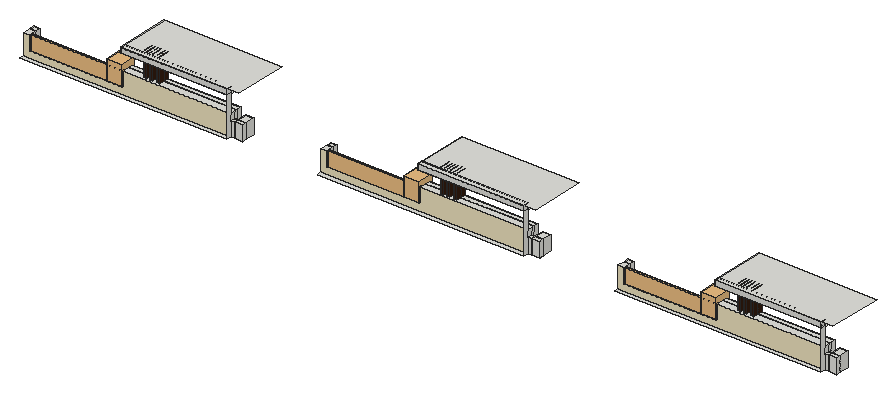
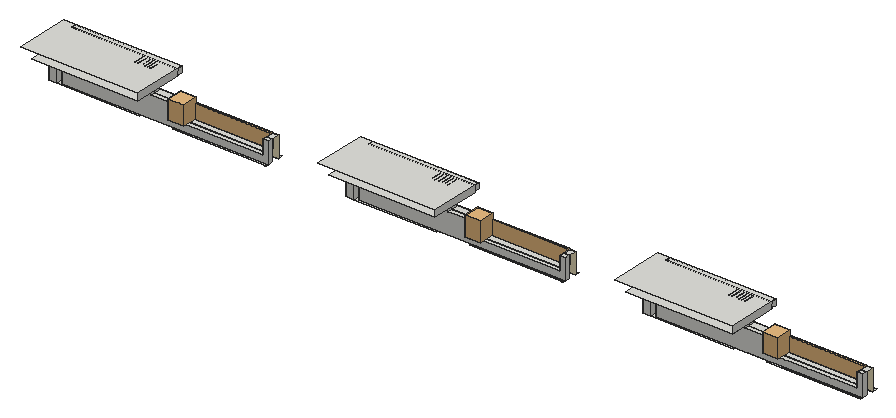
# SketchUp Ruby script. Lengths in inches.
U = 1.inch
M = Sketchup.active_model
def pt(a) = Geom::Point3d.new(a.map { |v| v * U })
def face(e, loops, mat)
  f = e.add_face(loops[0].map { |a| pt(a) })
  loops[1..].each { |l| e.add_face(l.map { |a| pt(a) }).erase! }
  f.material = f.back_material = mat if mat
  f
end
# faces: each face lists its corners as indices into pts; further lists are holes
def faces(e, pts, list, mat = nil) = list.each { |f| face(e, (f[0].is_a?(Array) ? f : [f]).map { |l| l.map { |i| pts[i] } }, mat) }
# xy, xz, yz: faces in a plane at the given z, y or x. An outline is a flat list of corners, or four numbers for a rectangle; further outlines are holes
def ring(l) = l.size == 4 ? [[l[0], l[1]], [l[2], l[1]], [l[2], l[3]], [l[0], l[3]]] : l.each_slice(2).to_a
def flat(e, list, mat, &to3) = list.each { |f| face(e, (f[0].is_a?(Array) ? f : [f]).map { |l| ring(l).map { |u, v| to3.(u, v) } }, mat) }
def xy(e, z, list, mat = nil) = flat(e, list, mat) { |x, y| [x, y, z] }
def xz(e, y, list, mat = nil) = flat(e, list, mat) { |x, z| [x, y, z] }
def yz(e, x, list, mat = nil) = flat(e, list, mat) { |y, z| [x, y, z] }
def lines(e, pts, list) = list.each { |a, b| e.add_line(pt(pts[a]), pt(pts[b])) }
# prism: a flat outline (further loops are holes) pulled along v
def prism(e, loops, v, mat = nil)
  f = face(e, loops, mat); d = Geom::Vector3d.new(v.map { |x| x * U })
  f.pushpull(f.normal.samedirection?(d) ? d.length : -d.length)
end
def box(e, o, s, mat = nil) = prism(e, [[o, [o[0] + s[0], o[1], o[2]], [o[0] + s[0], o[1] + s[1], o[2]], [o[0], o[1] + s[1], o[2]]]], [0, 0, s[2]], mat)
def at(x, y, z, deg = 0) = Geom::Transformation.translation(pt([x, y, z])) * Geom::Transformation.rotation(ORIGIN, Z_AXIS, deg.degrees)
def axes(o, x, y, z) = Geom::Transformation.new([*x, 0, *y, 0, *z, 0, *pt(o).to_a, 1])
def part(name) = M.definitions.add(name)
# library, detail: a bought-in or finely detailed component or shape, given as its bounding box
def library(name, o, s) = part(name).tap { |d| box(d.entities, o, s) }
def detail(e, o, s) = box(e.add_group.entities, o, s)
def put(e, d, t, mat = nil) = e.add_instance(d, t).tap { |i| i.material = mat if mat }
def group(e, t, mat = nil) = e.add_group.tap { |g| g.transformation = t; g.material = mat if mat }.entities
root = M.entities
M.materials.add("[Color D01]").color = [237, 225, 189]
M.materials.add("[Wood Veneer 01]").color = [51, 28, 15]
c1 = library("plant (1)",[-35.72,-28.42,0],[66.31,67.39,84.38])
c2 = library("Glass Railing",[0,0,0],[139.5,4.76,42])
xy(root,524.9375,[[83.125,246.64,593.4375,258.35],[816.6875,246.64,1327,258.35],[1550.25,246.64,2060.5625,258.35],[602.25,258.35,622,270.05],[622,258.35,622.125,270.05],
  [1335.8125,258.35,1355.5625,270.05],[1355.5625,258.35,1355.6875,270.05],[2069.375,258.35,2089.125,270.05],[2089.125,258.35,2089.25,270.05],[593.5,270.05,602.25,270.05,602.25,293.45,396.57,293.45,396.57,289.27,593.5,289.27],
  [602.25,270.05,622,293.45],[622,270.05,622.125,293.45],[1327.0625,270.05,1335.8125,270.05,1335.8125,293.45,1130.14,293.45,1130.14,289.27,1327.0625,289.27],[1335.8125,270.05,1355.5625,293.45],[1355.5625,270.05,1355.6875,293.45],
  [2060.625,270.05,2069.375,270.05,2069.375,293.45,1863.7,293.45,1863.7,289.27,2060.625,289.27],[2069.375,270.05,2089.125,293.45],[2089.125,270.05,2089.25,293.45],[318.81,271.96,322.23,277.39],[1052.37,271.96,1055.8,277.39],
  [1785.93,271.96,1789.36,277.39],[390.12,272.89,393.55,277.39],[1123.68,272.89,1127.11,277.39],[1857.25,272.89,1860.67,277.39],[83.125,277.39,318.81,277.39,318.81,286.21,315.43,286.21,315.43,289.27,83.125,289.27],
  [318.81,277.39,322.23,289.27],[322.23,277.39,322.23,286.21,324.81,286.21,324.81,282.52,328.23,282.52,328.23,286.21,330.81,286.21,330.81,282.52,334.23,282.52,334.23,286.21,336.81,286.21,336.81,282.52,340.23,282.52,340.23,286.21,342.81,286.21,342.81,282.52,346.23,282.52,346.23,286.21,348.81,286.21,348.81,283.46,352.23,283.46,352.23,286.21,354.81,286.21,354.81,283.46,358.23,283.46,358.23,286.21,360.81,286.21,360.81,283.46,364.23,283.46,364.23,286.21,366.81,286.21,366.81,283.46,370.23,283.46,370.23,286.21,372.81,286.21,372.81,283.46,376.23,283.46,376.23,286.21,378.81,286.21,378.81,283.46,382.23,283.46,382.23,286.21,384.81,286.21,384.81,283.46,388.23,283.46,388.23,286.21,390.12,286.21,390.12,277.39],[390.12,277.39,393.55,289.27],[393.55,277.39,593.5,277.39,593.5,289.27,396.57,289.27,396.57,286.21,393.55,286.21],[816.6875,277.39,1052.37,277.39,1052.37,286.21,1049,286.21,1049,289.27,816.6875,289.27],
  [1052.37,277.39,1055.8,289.27],[1055.8,277.39,1055.8,286.21,1058.37,286.21,1058.37,282.52,1061.8,282.52,1061.8,286.21,1064.37,286.21,1064.37,282.52,1067.8,282.52,1067.8,286.21,1070.37,286.21,1070.37,282.52,1073.8,282.52,1073.8,286.21,1076.37,286.21,1076.37,282.52,1079.8,282.52,1079.8,286.21,1082.37,286.21,1082.37,283.46,1085.8,283.46,1085.8,286.21,1088.37,286.21,1088.37,283.46,1091.8,283.46,1091.8,286.21,1094.37,286.21,1094.37,283.46,1097.8,283.46,1097.8,286.21,1100.37,286.21,1100.37,283.46,1103.8,283.46,1103.8,286.21,1106.37,286.21,1106.37,283.46,1109.8,283.46,1109.8,286.21,1112.37,286.21,1112.37,283.46,1115.8,283.46,1115.8,286.21,1118.37,286.21,1118.37,283.46,1121.8,283.46,1121.8,286.21,1123.68,286.21,1123.68,277.39],[1123.68,277.39,1127.11,289.27],[1127.11,277.39,1327.0625,277.39,1327.0625,289.27,1130.14,289.27,1130.14,286.21,1127.11,286.21],[1550.25,277.39,1785.93,277.39,1785.93,286.21,1782.56,286.21,1782.56,289.27,1550.25,289.27],
  [1785.93,277.39,1789.36,289.27],[1789.36,277.39,1789.36,286.21,1791.93,286.21,1791.93,282.52,1795.36,282.52,1795.36,286.21,1797.93,286.21,1797.93,282.52,1801.36,282.52,1801.36,286.21,1803.93,286.21,1803.93,282.52,1807.36,282.52,1807.36,286.21,1809.93,286.21,1809.93,282.52,1813.36,282.52,1813.36,286.21,1815.93,286.21,1815.93,283.46,1819.36,283.46,1819.36,286.21,1821.93,286.21,1821.93,283.46,1825.36,283.46,1825.36,286.21,1827.93,286.21,1827.93,283.46,1831.36,283.46,1831.36,286.21,1833.93,286.21,1833.93,283.46,1837.36,283.46,1837.36,286.21,1839.93,286.21,1839.93,283.46,1843.36,283.46,1843.36,286.21,1845.93,286.21,1845.93,283.46,1849.36,283.46,1849.36,286.21,1851.93,286.21,1851.93,283.46,1855.36,283.46,1855.36,286.21,1857.25,286.21,1857.25,277.39],[1857.25,277.39,1860.67,289.27],[1860.67,277.39,2060.625,277.39,2060.625,289.27,1863.7,289.27,1863.7,286.21,1860.67,286.21],[324.81,282.52,324.81,286.21,322.23,286.21,322.23,289.27,390.12,289.27,390.12,286.21,388.23,286.21,388.23,283.46,384.81,283.46,384.81,286.21,382.23,286.21,382.23,283.46,378.81,283.46,378.81,286.21,376.23,286.21,376.23,283.46,372.81,283.46,372.81,286.21,370.23,286.21,370.23,283.46,366.81,283.46,366.81,286.21,364.23,286.21,364.23,283.46,360.81,283.46,360.81,286.21,358.23,286.21,358.23,283.46,354.81,283.46,354.81,286.21,352.23,286.21,352.23,283.46,348.81,283.46,348.81,286.21,346.23,286.21,346.23,282.52,342.81,282.52,342.81,286.21,340.23,286.21,340.23,282.52,336.81,282.52,336.81,286.21,334.23,286.21,334.23,282.52,330.81,282.52,330.81,286.21,328.23,286.21,328.23,282.52],
  [1058.37,282.52,1058.37,286.21,1055.8,286.21,1055.8,289.27,1123.68,289.27,1123.68,286.21,1121.8,286.21,1121.8,283.46,1118.37,283.46,1118.37,286.21,1115.8,286.21,1115.8,283.46,1112.37,283.46,1112.37,286.21,1109.8,286.21,1109.8,283.46,1106.37,283.46,1106.37,286.21,1103.8,286.21,1103.8,283.46,1100.37,283.46,1100.37,286.21,1097.8,286.21,1097.8,283.46,1094.37,283.46,1094.37,286.21,1091.8,286.21,1091.8,283.46,1088.37,283.46,1088.37,286.21,1085.8,286.21,1085.8,283.46,1082.37,283.46,1082.37,286.21,1079.8,286.21,1079.8,282.52,1076.37,282.52,1076.37,286.21,1073.8,286.21,1073.8,282.52,1070.37,282.52,1070.37,286.21,1067.8,286.21,1067.8,282.52,1064.37,282.52,1064.37,286.21,1061.8,286.21,1061.8,282.52],[1791.93,282.52,1791.93,286.21,1789.36,286.21,1789.36,289.27,1857.25,289.27,1857.25,286.21,1855.36,286.21,1855.36,283.46,1851.93,283.46,1851.93,286.21,1849.36,286.21,1849.36,283.46,1845.93,283.46,1845.93,286.21,1843.36,286.21,1843.36,283.46,1839.93,283.46,1839.93,286.21,1837.36,286.21,1837.36,283.46,1833.93,283.46,1833.93,286.21,1831.36,286.21,1831.36,283.46,1827.93,283.46,1827.93,286.21,1825.36,286.21,1825.36,283.46,1821.93,283.46,1821.93,286.21,1819.36,286.21,1819.36,283.46,1815.93,283.46,1815.93,286.21,1813.36,286.21,1813.36,282.52,1809.93,282.52,1809.93,286.21,1807.36,286.21,1807.36,282.52,1803.93,282.52,1803.93,286.21,1801.36,286.21,1801.36,282.52,1797.93,282.52,1797.93,286.21,1795.36,286.21,1795.36,282.52],[315.43,286.21,318.81,289.27],[393.55,286.21,396.57,289.27],[1049,286.21,1052.37,289.27],
  [1127.11,286.21,1130.14,289.27],[1782.56,286.21,1785.93,289.27],[1860.67,286.21,1863.7,289.27],[83.125,289.27,315.43,293.46],[816.6875,289.27,1049,293.46],
  [1550.25,289.27,1782.56,293.46],[83.125,293.46,315.43,294.83],[816.6875,293.46,1049,294.83],[1550.25,293.46,1782.56,294.83]])
xy(root,541.61,[[97.01,258.35,324.51,277.39],[830.57,258.35,1058.07,277.39],[1564.13,258.35,1791.63,277.39],[97.01,277.39,324.51,289.27],[830.57,277.39,1058.07,289.27],
  [1564.13,277.39,1791.63,289.27]])
xy(root,560.9375,[[593.5,258.35,602.25,270.05],[602.25,258.35,622,270.05],[622,258.35,622.125,270.05],[1327.0625,258.35,1335.8125,270.05],[1335.8125,258.35,1355.5625,270.05],
  [1355.5625,258.35,1355.6875,270.05],[2060.625,258.35,2069.375,270.05],[2069.375,258.35,2089.125,270.05],[2089.125,258.35,2089.25,270.05],[602.25,270.05,622,293.45],
  [622,270.05,622.125,293.45],[1335.8125,270.05,1355.5625,293.45],[1355.5625,270.05,1355.6875,293.45],[2069.375,270.05,2089.125,293.45],[2089.125,270.05,2089.25,293.45]])
xy(root,576.8125,[[83.125,258.35,97.01,277.39],[324.51,258.35,593.5,258.35,593.5,277.39,413.09,277.39,413.09,264.45,405.09,264.45,405.09,277.39,396.02,277.39,396.02,264.45,388.02,264.45,388.02,277.39,381.65,277.39,381.65,264.45,373.65,264.45,373.65,277.39,324.51,277.39],[816.6875,258.35,830.57,277.39],[1058.07,258.35,1327.0625,258.35,1327.0625,277.39,1146.65,277.39,1146.65,264.45,1138.65,264.45,1138.65,277.39,1129.59,277.39,1129.59,264.45,1121.59,264.45,1121.59,277.39,1115.21,277.39,1115.21,264.45,1107.21,264.45,1107.21,277.39,1058.07,277.39],[1550.25,258.35,1564.13,277.39],
  [1791.63,258.35,2060.625,258.35,2060.625,277.39,1880.21,277.39,1880.21,264.45,1872.21,264.45,1872.21,277.39,1863.15,277.39,1863.15,264.45,1855.15,264.45,1855.15,277.39,1848.77,277.39,1848.77,264.45,1840.77,264.45,1840.77,277.39,1791.63,277.39],[83.125,277.39,97.01,289.27],[324.51,277.39,373.65,289.27],[381.65,277.39,388.02,289.27],[396.02,277.39,405.09,289.27],
  [413.09,277.39,593.5,289.27],[816.6875,277.39,830.57,289.27],[1058.07,277.39,1107.21,289.27],[1115.21,277.39,1121.59,289.27],[1129.59,277.39,1138.65,289.27],
  [1146.65,277.39,1327.0625,289.27],[1550.25,277.39,1564.13,289.27],[1791.63,277.39,1840.77,289.27],[1848.77,277.39,1855.15,289.27],[1863.15,277.39,1872.21,289.27],
  [1880.21,277.39,2060.625,289.27]])
xy(root,620.22,[[330.81,258.35,593.5,381.35],[1064.37,258.35,1327.0625,381.35],[1797.93,258.35,2060.625,381.35]])
xy(root,635.84,[[373.65,264.45,381.65,277.39],[388.02,264.45,396.02,277.39],[405.09,264.45,413.09,277.39],[1107.21,264.45,1115.21,277.39],[1121.59,264.45,1129.59,277.39],
  [1138.65,264.45,1146.65,277.39],[1840.77,264.45,1848.77,277.39],[1855.15,264.45,1863.15,277.39],[1872.21,264.45,1880.21,277.39],[373.65,277.39,381.65,289.27],
  [388.02,277.39,396.02,289.27],[405.09,277.39,413.09,289.27],[1107.21,277.39,1115.21,289.27],[1121.59,277.39,1129.59,289.27],[1138.65,277.39,1146.65,289.27],
  [1840.77,277.39,1848.77,289.27],[1855.15,277.39,1863.15,289.27],[1872.21,277.39,1880.21,289.27]])
xy(root,636.53,[[330.81,246.64,622,381.35],[1064.37,246.64,1355.5625,381.35],[1797.93,246.64,2089.125,381.35]])
xz(root,258.35,[[593.4375,524.9375,602.25,524.9375,602.25,560.9375,593.5,560.9375,593.5,576.8125,593.4375,576.8125],[602.25,524.9375,622,560.9375],[622,524.9375,622.125,560.9375],[1327,524.9375,1335.8125,524.9375,1335.8125,560.9375,1327.0625,560.9375,1327.0625,576.8125,1327,576.8125],[1335.8125,524.9375,1355.5625,560.9375],
  [1355.5625,524.9375,1355.6875,560.9375],[2060.5625,524.9375,2069.375,524.9375,2069.375,560.9375,2060.625,560.9375,2060.625,576.8125,2060.5625,576.8125],[2069.375,524.9375,2089.125,560.9375],[2089.125,524.9375,2089.25,560.9375],[593.4375,576.8125,593.5,620.22],
  [1327,576.8125,1327.0625,620.22],[2060.5625,576.8125,2060.625,620.22],[330.81,620.22,593.4375,620.22,593.4375,623.82,593.5,623.82,593.5,636.53,330.81,636.53],[1064.37,620.22,1327,620.22,1327,623.82,1327.0625,623.82,1327.0625,636.53,1064.37,636.53],[1797.93,620.22,2060.5625,620.22,2060.5625,623.82,2060.625,623.82,2060.625,636.53,1797.93,636.53]])
xz(root,258.35,[[83.125,524.9375,593.4375,524.9375,593.4375,576.8125,324.51,576.8125,324.51,541.61,97.01,541.61,97.01,576.8125,83.125,576.8125],[816.6875,524.9375,1327,524.9375,1327,576.8125,1058.07,576.8125,1058.07,541.61,830.57,541.61,830.57,576.8125,816.6875,576.8125],[1550.25,524.9375,2060.5625,524.9375,2060.5625,576.8125,1791.63,576.8125,1791.63,541.61,1564.13,541.61,1564.13,576.8125,1550.25,576.8125]],"[Color D01]")
xz(root,264.45,[[373.65,576.8125,381.65,635.84],[388.02,576.8125,396.02,635.84],[405.09,576.8125,413.09,635.84],[1107.21,576.8125,1115.21,635.84],[1121.59,576.8125,1129.59,635.84],
  [1138.65,576.8125,1146.65,635.84],[1840.77,576.8125,1848.77,635.84],[1855.15,576.8125,1863.15,635.84],[1872.21,576.8125,1880.21,635.84]],"[Wood Veneer 01]")
xz(root,270.05,[[593.5,524.9375,602.25,560.9375],[602.25,524.9375,622.125,560.9375],[1327.0625,524.9375,1335.8125,560.9375],[1335.8125,524.9375,1355.6875,560.9375],[2060.625,524.9375,2069.375,560.9375],
  [2069.375,524.9375,2089.25,560.9375]])
xz(root,277.39,[[83.125,524.9375,593.5,524.9375,593.5,576.8125,413.09,576.8125,413.09,635.84,405.09,635.84,405.09,576.8125,396.02,576.8125,396.02,635.84,388.02,635.84,388.02,576.8125,381.65,576.8125,381.65,635.84,373.65,635.84,373.65,576.8125,324.51,576.8125,324.51,541.61,97.01,541.61,97.01,576.8125,83.125,576.8125],[816.6875,524.9375,1327.0625,524.9375,1327.0625,576.8125,1146.65,576.8125,1146.65,635.84,1138.65,635.84,1138.65,576.8125,1129.59,576.8125,1129.59,635.84,1121.59,635.84,1121.59,576.8125,1115.21,576.8125,1115.21,635.84,1107.21,635.84,1107.21,576.8125,1058.07,576.8125,1058.07,541.61,830.57,541.61,830.57,576.8125,816.6875,576.8125],[1550.25,524.9375,2060.625,524.9375,2060.625,576.8125,1880.21,576.8125,1880.21,635.84,1872.21,635.84,1872.21,576.8125,1863.15,576.8125,1863.15,635.84,1855.15,635.84,1855.15,576.8125,1848.77,576.8125,1848.77,635.84,1840.77,635.84,1840.77,576.8125,1791.63,576.8125,1791.63,541.61,1564.13,541.61,1564.13,576.8125,1550.25,576.8125]])
xz(root,289.27,[[83.125,524.9375,83.125,576.8125,97.01,576.8125,97.01,541.61,324.51,541.61,324.51,576.8125,373.65,576.8125,373.65,635.84,381.65,635.84,381.65,576.8125,388.02,576.8125,388.02,635.84,396.02,635.84,396.02,576.8125,405.09,576.8125,405.09,635.84,413.09,635.84,413.09,576.8125,593.5,576.8125,593.5,524.9375],[816.6875,524.9375,816.6875,576.8125,830.57,576.8125,830.57,541.61,1058.07,541.61,1058.07,576.8125,1107.21,576.8125,1107.21,635.84,1115.21,635.84,1115.21,576.8125,1121.59,576.8125,1121.59,635.84,1129.59,635.84,1129.59,576.8125,1138.65,576.8125,1138.65,635.84,1146.65,635.84,1146.65,576.8125,1327.0625,576.8125,1327.0625,524.9375],[1550.25,524.9375,1550.25,576.8125,1564.13,576.8125,1564.13,541.61,1791.63,541.61,1791.63,576.8125,1840.77,576.8125,1840.77,635.84,1848.77,635.84,1848.77,576.8125,1855.15,576.8125,1855.15,635.84,1863.15,635.84,1863.15,576.8125,1872.21,576.8125,1872.21,635.84,1880.21,635.84,1880.21,576.8125,2060.625,576.8125,2060.625,524.9375]])
xz(root,293.45,[[602.25,524.9375,622,560.9375],[622,524.9375,622.125,560.9375],[1335.8125,524.9375,1355.5625,560.9375],[1355.5625,524.9375,1355.6875,560.9375],[2069.375,524.9375,2089.125,560.9375],
  [2089.125,524.9375,2089.25,560.9375]])
yz(root,83.125,[[277.39,524.9375,289.27,576.8125]])
yz(root,97.01,[[258.35,541.61,277.39,576.8125],[277.39,541.61,289.27,576.8125]])
yz(root,324.51,[[258.35,541.61,277.39,576.8125],[277.39,541.61,289.27,576.8125]])
yz(root,330.81,[[258.35,620.22,258.35,623.82,259.1,623.87,258.35,636.53,246.64,635.84,246.64,636.53,381.35,636.53,381.35,620.22],[247.39,623.17,246.64,635.84,258.35,636.53,258.35,623.82],[258.35,623.82,258.35,636.53,259.1,623.87]])
yz(root,373.65,[[264.45,576.8125,277.39,635.84],[277.39,576.8125,289.27,635.84]])
yz(root,381.65,[[277.39,576.8125,289.27,635.84]])
yz(root,381.65,[[264.45,576.8125,277.39,635.84]],"[Wood Veneer 01]")
yz(root,388.02,[[264.45,576.8125,277.39,635.84],[277.39,576.8125,289.27,635.84]])
yz(root,396.02,[[264.45,576.8125,277.39,635.84],[277.39,576.8125,289.27,635.84]],"[Wood Veneer 01]")
yz(root,405.09,[[264.45,576.8125,277.39,635.84],[277.39,576.8125,289.27,635.84]])
yz(root,413.09,[[264.45,576.8125,277.39,635.84],[277.39,576.8125,289.27,635.84]],"[Wood Veneer 01]")
yz(root,593.4375,[[246.64,524.9375,246.64,635.84,247.39,623.17,258.35,623.82,258.35,524.9375]])
yz(root,593.5,[[270.05,524.9375,277.39,576.8125],[277.39,524.9375,289.27,576.8125],[258.35,560.9375,270.05,576.8125],[247.39,623.17,246.64,635.84,258.35,636.53,258.35,623.82],[258.35,623.82,259.1,623.87,258.35,636.53]])
yz(root,602.25,[[258.35,524.9375,270.05,560.9375],[270.05,524.9375,293.45,560.9375]])
yz(root,622.125,[[258.35,524.9375,270.05,560.9375],[270.05,524.9375,293.45,560.9375]])
yz(root,816.6875,[[277.39,524.9375,289.27,576.8125]])
yz(root,830.57,[[258.35,541.61,277.39,576.8125],[277.39,541.61,289.27,576.8125]])
yz(root,1058.07,[[258.35,541.61,277.39,576.8125],[277.39,541.61,289.27,576.8125]])
yz(root,1064.37,[[258.35,620.22,258.35,623.82,259.1,623.87,258.35,636.53,246.64,635.84,246.64,636.53,381.35,636.53,381.35,620.22],[247.39,623.17,246.64,635.84,258.35,636.53,258.35,623.82],[258.35,623.82,258.35,636.53,259.1,623.87]])
yz(root,1107.21,[[264.45,576.8125,277.39,635.84],[277.39,576.8125,289.27,635.84]])
yz(root,1115.21,[[277.39,576.8125,289.27,635.84]])
yz(root,1115.21,[[264.45,576.8125,277.39,635.84]],"[Wood Veneer 01]")
yz(root,1121.59,[[264.45,576.8125,277.39,635.84],[277.39,576.8125,289.27,635.84]])
yz(root,1129.59,[[264.45,576.8125,277.39,635.84],[277.39,576.8125,289.27,635.84]],"[Wood Veneer 01]")
yz(root,1138.65,[[264.45,576.8125,277.39,635.84],[277.39,576.8125,289.27,635.84]])
yz(root,1146.65,[[264.45,576.8125,277.39,635.84],[277.39,576.8125,289.27,635.84]],"[Wood Veneer 01]")
yz(root,1327,[[246.64,524.9375,246.64,635.84,247.39,623.17,258.35,623.82,258.35,524.9375]])
yz(root,1327.0625,[[270.05,524.9375,277.39,576.8125],[277.39,524.9375,289.27,576.8125],[258.35,560.9375,270.05,576.8125],[247.39,623.17,246.64,635.84,258.35,636.53,258.35,623.82],[258.35,623.82,259.1,623.87,258.35,636.53]])
yz(root,1335.8125,[[258.35,524.9375,270.05,560.9375],[270.05,524.9375,293.45,560.9375]])
yz(root,1355.6875,[[258.35,524.9375,270.05,560.9375],[270.05,524.9375,293.45,560.9375]])
yz(root,1550.25,[[277.39,524.9375,289.27,576.8125]])
yz(root,1564.13,[[258.35,541.61,277.39,576.8125],[277.39,541.61,289.27,576.8125]])
yz(root,1791.63,[[258.35,541.61,277.39,576.8125],[277.39,541.61,289.27,576.8125]])
yz(root,1797.93,[[258.35,620.22,258.35,623.82,259.1,623.87,258.35,636.53,246.64,635.84,246.64,636.53,381.35,636.53,381.35,620.22],[247.39,623.17,246.64,635.84,258.35,636.53,258.35,623.82],[258.35,623.82,258.35,636.53,259.1,623.87]])
yz(root,1840.77,[[264.45,576.8125,277.39,635.84],[277.39,576.8125,289.27,635.84]])
yz(root,1848.77,[[277.39,576.8125,289.27,635.84]])
yz(root,1848.77,[[264.45,576.8125,277.39,635.84]],"[Wood Veneer 01]")
yz(root,1855.15,[[264.45,576.8125,277.39,635.84],[277.39,576.8125,289.27,635.84]])
yz(root,1863.15,[[264.45,576.8125,277.39,635.84],[277.39,576.8125,289.27,635.84]],"[Wood Veneer 01]")
yz(root,1872.21,[[264.45,576.8125,277.39,635.84],[277.39,576.8125,289.27,635.84]])
yz(root,1880.21,[[264.45,576.8125,277.39,635.84],[277.39,576.8125,289.27,635.84]],"[Wood Veneer 01]")
yz(root,2060.5625,[[246.64,524.9375,246.64,635.84,247.39,623.17,258.35,623.82,258.35,524.9375]])
yz(root,2060.625,[[270.05,524.9375,277.39,576.8125],[277.39,524.9375,289.27,576.8125],[258.35,560.9375,270.05,576.8125],[247.39,623.17,246.64,635.84,258.35,636.53,258.35,623.82],[258.35,623.82,259.1,623.87,258.35,636.53]])
yz(root,2069.375,[[258.35,524.9375,270.05,560.9375],[270.05,524.9375,293.45,560.9375]])
yz(root,2089.25,[[258.35,524.9375,270.05,560.9375],[270.05,524.9375,293.45,560.9375]])
p = [[330.81,247.39,623.17],[593.4375,247.39,623.17],[593.4375,246.64,635.84],[330.81,246.64,635.84],[593.5,247.39,623.17],[593.5,246.64,635.84],
  [1064.37,247.39,623.17],[1327,247.39,623.17],[1327,246.64,635.84],[1064.37,246.64,635.84],[1327.0625,247.39,623.17],[1327.0625,246.64,635.84],
  [1797.93,247.39,623.17],[2060.5625,247.39,623.17],[2060.5625,246.64,635.84],[1797.93,246.64,635.84],[2060.625,247.39,623.17],[2060.625,246.64,635.84],
  [593.5,259.1,623.87],[593.5,258.35,623.82],[593.4375,258.35,623.82],[330.81,258.35,623.82],[330.81,259.1,623.87],[1327.0625,259.1,623.87],
  [1327.0625,258.35,623.82],[1327,258.35,623.82],[1064.37,258.35,623.82],[1064.37,259.1,623.87],[2060.625,259.1,623.87],[2060.625,258.35,623.82],
  [2060.5625,258.35,623.82],[1797.93,258.35,623.82],[1797.93,259.1,623.87],[330.81,258.35,636.53],[593.5,258.35,636.53],[1064.37,258.35,636.53],
  [1327.0625,258.35,636.53],[1797.93,258.35,636.53],[2060.625,258.35,636.53]]
faces(root,p,[[0,1,2,3],[4,5,2,1],[6,7,8,9],[10,11,8,7],[12,13,14,15],[16,17,14,13],[18,19,20,1,0,21,22],[19,4,1,20],
  [23,24,25,7,6,26,27],[24,10,7,25],[28,29,30,13,12,31,32],[29,16,13,30],[33,34,18,22],[35,36,23,27],[37,38,28,32],[5,34,33,3,2],
  [11,36,35,9,8],[17,38,37,15,14]])
put(root,c1,axes([1040.64,274.55,541.61],[0.57,0,0],[0,0.57,0],[0,0,0.57]))
put(root,c1,axes([1774.2,274.55,541.61],[0.57,0,0],[0,0.57,0],[0,0,0.57]))
put(root,c1,axes([307.08,274.55,541.61],[0.57,0,0],[0,0.57,0],[0,0,0.57]))
put(root,c2,axes([833.74,258.42,542.59],[1.62093,0,0],[0,0.83,0],[0,0,0.84]))
put(root,c2,axes([1567.3,258.42,542.59],[1.62093,0,0],[0,0.83,0],[0,0,0.84]))
put(root,c2,axes([100.18,258.42,542.59],[1.62093,0,0],[0,0.83,0],[0,0,0.84]))
